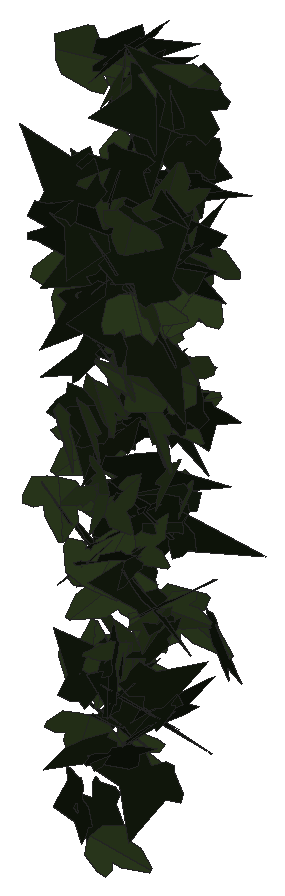
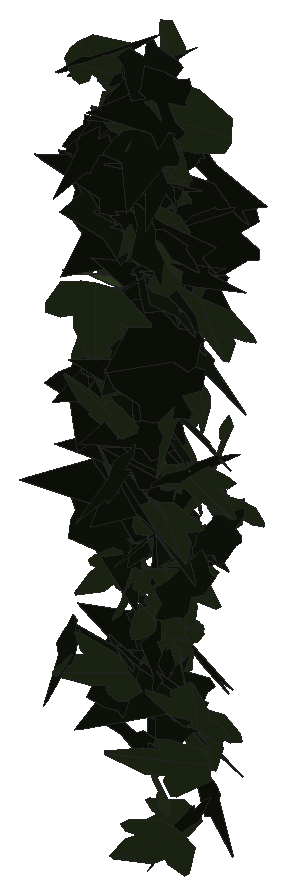
# SketchUp Ruby script. Lengths in inches.
U = 1.inch
M = Sketchup.active_model
def pt(a) = Geom::Point3d.new(a.map { |v| v * U })
def face(e, loops, mat)
  f = e.add_face(loops[0].map { |a| pt(a) })
  loops[1..].each { |l| e.add_face(l.map { |a| pt(a) }).erase! }
  f.material = f.back_material = mat if mat
  f
end
# faces: each face lists its corners as indices into pts; further lists are holes
def faces(e, pts, list, mat = nil) = list.each { |f| face(e, (f[0].is_a?(Array) ? f : [f]).map { |l| l.map { |i| pts[i] } }, mat) }
# xy, xz, yz: faces in a plane at the given z, y or x. An outline is a flat list of corners, or four numbers for a rectangle; further outlines are holes
def ring(l) = l.size == 4 ? [[l[0], l[1]], [l[2], l[1]], [l[2], l[3]], [l[0], l[3]]] : l.each_slice(2).to_a
def flat(e, list, mat, &to3) = list.each { |f| face(e, (f[0].is_a?(Array) ? f : [f]).map { |l| ring(l).map { |u, v| to3.(u, v) } }, mat) }
def xy(e, z, list, mat = nil) = flat(e, list, mat) { |x, y| [x, y, z] }
def xz(e, y, list, mat = nil) = flat(e, list, mat) { |x, z| [x, y, z] }
def yz(e, x, list, mat = nil) = flat(e, list, mat) { |y, z| [x, y, z] }
def lines(e, pts, list) = list.each { |a, b| e.add_line(pt(pts[a]), pt(pts[b])) }
# prism: a flat outline (further loops are holes) pulled along v
def prism(e, loops, v, mat = nil)
  f = face(e, loops, mat); d = Geom::Vector3d.new(v.map { |x| x * U })
  f.pushpull(f.normal.samedirection?(d) ? d.length : -d.length)
end
def box(e, o, s, mat = nil) = prism(e, [[o, [o[0] + s[0], o[1], o[2]], [o[0] + s[0], o[1] + s[1], o[2]], [o[0], o[1] + s[1], o[2]]]], [0, 0, s[2]], mat)
def at(x, y, z, deg = 0) = Geom::Transformation.translation(pt([x, y, z])) * Geom::Transformation.rotation(ORIGIN, Z_AXIS, deg.degrees)
def axes(o, x, y, z) = Geom::Transformation.new([*x, 0, *y, 0, *z, 0, *pt(o).to_a, 1])
def part(name) = M.definitions.add(name)
# library, detail: a bought-in or finely detailed component or shape, given as its bounding box
def library(name, o, s) = part(name).tap { |d| box(d.entities, o, s) }
def detail(e, o, s) = box(e.add_group.entities, o, s)
def put(e, d, t, mat = nil) = e.add_instance(d, t).tap { |i| i.material = mat if mat }
def group(e, t, mat = nil) = e.add_group.tap { |g| g.transformation = t; g.material = mat if mat }.entities
root = M.entities
M.materials.add("1026 AP 7946 SUNNY SIDE UP").color = [254, 231, 186]
M.materials.add("efeu1").color = [18, 25, 13]
M.materials.add("efeu2").color = [43, 57, 29]
c1 = part("ivyleaf_10")
p = [[0,0.5,-0.03],[-0.0625,2.02,-0.43],[-0.19,2.01,-0.46],[-0.54,1.05,-0.29],[-0.52,0.625,-0.18],[-0.83,0.76,-0.28],
  [-1.16,0.64,-0.33],[-1.15,0.33,-0.24],[-0.77,-0.39,0.02],[-0.3,-0.51,0.16],[0.04,-0.48,0.23],[-0.02,2.01,-0.4375],
  [-0.06,2.01,-0.43],[0.04,-0.49,0.23],[0.67,-0.49,0.14],[1.38,0.36,-0.2],[1.375,0.51,-0.24],[0.81,0.65,-0.19],
  [0.62,0.59,-0.15],[0.6,1.09,-0.28],[0.5,1.23,-0.31]]
faces(c1.entities,p,[[0,1,2,3,4,5,6,7,8,9,10],[11,12,0,13,14,15,16,17,18,19,20]],"efeu2")
c2 = part("ivyleaf_9")
p = [[1.54,2.16,1.25],[1.36,2.04,1.19],[-0.21,0.99,0.68],[-0.71,1.11,0.82],[-0.85,0.86,0.67],[-0.8,0.17,0.21],
  [-0.9,-0.01,0.1],[-0.67,-0.16,-0.02],[-0.08,-0.08,-0.05],[-0.03,-0.6,-0.4],[0.65,-0.88,-0.66],[0.83,-0.6,-0.49],
  [1.29,-0.42,-0.43],[1.8125,-0.07,-0.26],[1.21,0.44,0.15]]
faces(c2.entities,p,[[0,1,2,3,4,5,6,7,8,9,10,11,12,13,14]],"efeu1")
put(root,c1,axes([136.21,211.66,278.86],[-0.0278,-0.0094,0.38094],[0.4911,0.19805,0.02172],[-0.31176,0.31282,0.00025]),"1026 AP 7946 SUNNY SIDE UP")
put(root,c2,axes([136.35,211.04,272.625],[0.38727,-0.21719,0.00095],[-0.02228,-0.01932,-0.33751],[0.3408,0.24554,-0.02314]),"1026 AP 7946 SUNNY SIDE UP")
put(root,c1,axes([136.59,210.88,273.87],[-0.17293,0.2877,-0.01409],[-0.00417,-0.0174,-0.31728],[-0.453,-0.10967,0.0083]),"1026 AP 7946 SUNNY SIDE UP")
put(root,c2,axes([137,210.68,277.4375],[-0.06506,0.1165,0.38031],[-0.30524,0.3142,-0.12295],[-0.52547,-0.19694,0.02433]),"1026 AP 7946 SUNNY SIDE UP")
put(root,c1,axes([136.59,211.27,275.9],[0.62304,-0.07737,0.00351],[-0.00388,-0.03262,-0.41475],[0.12175,0.39491,-0.03116]),"1026 AP 7946 SUNNY SIDE UP")
put(root,c1,axes([136.24,212.09,269.64],[0.01205,-0.08359,-0.38142],[0.5698,0.11024,-0.01729],[0.17508,-0.35303,0.08253]),"1026 AP 7946 SUNNY SIDE UP")
put(root,c1,axes([136.81,211.36,273.42],[0.43287,0.00126,-0.17753],[-0.27028,-0.02157,-0.28315],[-0.01967,0.32407,-0.01625]),"1026 AP 7946 SUNNY SIDE UP")
put(root,c2,axes([136.6,211.65,273.69],[-0.15607,-0.3225,0.05031],[-0.00558,-0.05189,-0.34771],[0.51329,-0.09862,0.01152]),"1026 AP 7946 SUNNY SIDE UP")
put(root,c1,axes([136.65,211.44,269.83],[0.56701,-0.03279,0.03863],[-0.0537,0.03854,0.37149],[-0.05731,-0.36051,0.03405]),"1026 AP 7946 SUNNY SIDE UP")
put(root,c1,axes([136.55,210.85,272.87],[0.46298,0.02912,0.08105],[0.12709,-0.02385,-0.30332],[-0.0344,0.3038,-0.02978]),"1026 AP 7946 SUNNY SIDE UP")
put(root,c1,axes([136.84,211.68,274.29],[-0.12414,0.22374,0.25419],[-0.18212,0.21792,-0.24173],[-0.48947,-0.13783,0.02547]),"1026 AP 7946 SUNNY SIDE UP")
put(root,c1,axes([136.53,212.18,268.47],[-0.32013,-0.08956,-0.24599],[0.38005,0.0277,-0.22332],[0.12556,-0.31218,0.04876]),"1026 AP 7946 SUNNY SIDE UP")
put(root,c2,axes([137.02,210.75,268.48],[0.05935,-0.02328,-0.31384],[-0.47182,0.05429,-0.04227],[0.08938,0.302,-0.01476]),"1026 AP 7946 SUNNY SIDE UP")
put(root,c2,axes([136.87,212.02,277.1],[0.06338,0.09978,0.33652],[0.08739,0.32205,-0.10671],[-0.52904,0.06515,0.02269]),"1026 AP 7946 SUNNY SIDE UP")
put(root,c2,axes([137.17,211.42,276.84],[-0.47664,0.02506,-0.15601],[-0.23934,-0.00342,0.31298],[0.03283,0.3389,0.01669]),"1026 AP 7946 SUNNY SIDE UP")
put(root,c2,axes([137.05,210.97,275.02],[-0.30513,0.21423,-0.02605],[0.0044,-0.03314,-0.29725],[-0.33939,-0.19303,0.01957]),"1026 AP 7946 SUNNY SIDE UP")
put(root,c1,axes([136.78,211.96,268.94],[0.31067,-0.25014,0.05999],[-0.03001,0.06076,0.32793],[-0.40323,-0.19724,0.02182]),"1026 AP 7946 SUNNY SIDE UP")
put(root,c1,axes([136.85,211.7,276.52],[0.12673,-0.28952,0.14914],[-0.03583,0.14544,0.31005],[-0.50888,-0.08234,0.01531]),"1026 AP 7946 SUNNY SIDE UP")
put(root,c2,axes([136.95,211.98,278.58],[0.39065,0.09106,-0.21504],[-0.3587,0.09027,-0.23802],[-0.01024,0.31203,0.13374]),"1026 AP 7946 SUNNY SIDE UP")
put(root,c2,axes([137.14,211.5,276.35],[-0.4536,-0.14948,0.15217],[-0.16699,-0.11441,-0.33172],[0.28623,-0.30364,0.04762]),"1026 AP 7946 SUNNY SIDE UP")
put(root,c2,axes([137.27,210.73,270.4],[-0.32936,0.03673,-0.25687],[-0.37724,0.07113,0.21866],[0.12245,0.31794,-0.01726]),"1026 AP 7946 SUNNY SIDE UP")
put(root,c2,axes([137.22,211.02,273.99],[-0.18833,0.21393,0.14502],[-0.16489,0.09937,-0.24905],[-0.36623,-0.15475,0.03755]),"1026 AP 7946 SUNNY SIDE UP")
put(root,c1,axes([136.99,210.89,269.5],[0.45851,0.0798,-0.05094],[-0.11625,0.09365,-0.2902],[-0.09159,0.28062,0.11329]),"1026 AP 7946 SUNNY SIDE UP")
put(root,c2,axes([136.65,211.57,271.76],[0.16872,-0.25415,0.21875],[0.16955,-0.18584,-0.28443],[0.49392,0.15061,0.02291]),"1026 AP 7946 SUNNY SIDE UP")
put(root,c2,axes([136.72,211.74,279],[0.21121,0.10646,0.30666],[0.3911,0.16298,-0.17508],[-0.30537,0.28237,-0.01213]),"1026 AP 7946 SUNNY SIDE UP")
put(root,c2,axes([136.54,210.75,276.83],[0.3807,0.08624,0.32324],[0.48957,0.05017,-0.26183],[-0.14614,0.39274,-0.03508]),"1026 AP 7946 SUNNY SIDE UP")
put(root,c2,axes([137.02,211.08,276.97],[-0.21776,-0.27597,0.09324],[-0.04613,-0.0882,-0.31833],[0.45511,-0.14098,0.01234]),"1026 AP 7946 SUNNY SIDE UP")
put(root,c2,axes([136.93,211.15,268.26],[0.19666,-0.20548,-0.23147],[-0.17736,0.19299,-0.24667],[0.44323,0.16839,0.004]),"1026 AP 7946 SUNNY SIDE UP")
put(root,c2,axes([137.22,211.36,276.01],[-0.34779,0.18257,-0.17716],[-0.17893,0.13283,0.29504],[0.3527,0.24741,-0.02502]),"1026 AP 7946 SUNNY SIDE UP")
put(root,c1,axes([137.17,211.39,275.76],[-0.10162,-0.08496,-0.34058],[-0.20899,-0.30312,0.10541],[-0.49357,0.14584,0.02549]),"1026 AP 7946 SUNNY SIDE UP")
put(root,c2,axes([137.24,211.01,275.89],[-0.00839,0.12717,-0.33309],[-0.00489,-0.3241,-0.13288],[-0.54736,0.00095,0.00629]),"1026 AP 7946 SUNNY SIDE UP")
put(root,c2,axes([137.3125,210.88,269.44],[-0.40724,0.14508,-0.03945],[0.03144,-0.04399,-0.30468],[-0.23417,-0.25821,0.0277]),"1026 AP 7946 SUNNY SIDE UP")
put(root,c2,axes([136.89,211.56,275.63],[0.42135,0.16585,0.0927],[0.14518,0.01918,-0.32296],[-0.25794,0.28172,-0.03035]),"1026 AP 7946 SUNNY SIDE UP")
put(root,c1,axes([137.02,210.83,274.2],[-0.25279,0.2106,-0.11458],[0.08724,-0.09886,-0.27311],[-0.36509,-0.16944,0.01407]),"1026 AP 7946 SUNNY SIDE UP")
put(root,c2,axes([137.28,211.34,276.1875],[-0.16919,0.29544,-0.13858],[0.0653,-0.1298,-0.32464],[-0.50735,-0.11523,0.00443]),"1026 AP 7946 SUNNY SIDE UP")
put(root,c2,axes([137.3,211.63,279.49],[-0.1922,0.29357,-0.15385],[0.05646,-0.14825,-0.32772],[-0.51602,-0.12557,0.02145]),"1026 AP 7946 SUNNY SIDE UP")
put(root,c1,axes([137.32,211.29,272.59],[-0.4199,-0.03014,0.13696],[-0.20203,-0.04319,-0.27585],[0.07241,-0.29524,0.02459]),"1026 AP 7946 SUNNY SIDE UP")
put(root,c1,axes([137.21,211.23,271.65],[0.42787,0.09204,-0.08743],[-0.17297,0.07655,-0.27569],[-0.09515,0.27473,0.10802]),"1026 AP 7946 SUNNY SIDE UP")
put(root,c1,axes([137.13,211.02,274.47],[-0.37343,0.1467,-0.05677],[0.04242,-0.06179,-0.2853],[-0.24319,-0.23603,0.0374]),"1026 AP 7946 SUNNY SIDE UP")
put(root,c1,axes([137.16,210.89,273.06],[-0.24187,-0.22442,-0.06813],[0.07849,0.04429,-0.27956],[0.35883,-0.16095,0.01523]),"1026 AP 7946 SUNNY SIDE UP")
put(root,c2,axes([137.15,211.02,269.72],[0.39357,0.0604,-0.15173],[-0.24928,0.06394,-0.24958],[-0.02762,0.28347,0.09045]),"1026 AP 7946 SUNNY SIDE UP")
put(root,c2,axes([137.33,210.89,272.32],[-0.2468,0.1555,-0.16482],[0.10857,-0.15326,-0.22291],[-0.33465,-0.1644,0.04924]),"1026 AP 7946 SUNNY SIDE UP")
put(root,c1,axes([137.33,211.03,271.64],[0.38389,0.09192,-0.19377],[-0.26093,-0.09249,-0.26826],[-0.20189,0.29432,-0.02173]),"1026 AP 7946 SUNNY SIDE UP")
put(root,c1,axes([137.39,210.7,273.2],[0.14032,-0.20353,-0.31049],[-0.19878,0.27235,-0.22732],[0.53458,0.1547,-0.00303]),"1026 AP 7946 SUNNY SIDE UP")
put(root,c1,axes([137.27,211.84,278.52],[0.51588,0.08091,0.08567],[-0.13834,0.01298,0.34656],[0.11814,-0.3381,0.03172]),"1026 AP 7946 SUNNY SIDE UP")
put(root,c2,axes([136.77,211.66,274.76],[0.27452,-0.01959,0.31551],[0.47403,-0.05567,-0.18097],[0.09123,0.34821,-0.00908]),"1026 AP 7946 SUNNY SIDE UP")
put(root,c2,axes([137.49,211.01,272.21],[-0.06595,0.25632,0.17768],[-0.14759,0.15376,-0.26024],[-0.46148,-0.08581,0.05784]),"1026 AP 7946 SUNNY SIDE UP")
put(root,c2,axes([137.32,211.31,273.99],[-0.42081,0.10903,-0.20635],[0.27057,-0.10758,-0.29689],[-0.23664,-0.31689,0.0275]),"1026 AP 7946 SUNNY SIDE UP")
put(root,c2,axes([137.47,211.1,277.96],[-0.08719,0.05467,-0.46596],[-0.52622,0.30475,0.08194],[0.48682,0.33921,0.00512]),"1026 AP 7946 SUNNY SIDE UP")
put(root,c2,axes([137.14,211.74,277.08],[-0.34262,-0.11414,-0.24567],[0.35966,0.07191,-0.25103],[0.20663,-0.31443,0.02959]),"1026 AP 7946 SUNNY SIDE UP")
put(root,c2,axes([137.32,210.9,272.39],[0.1511,0.23477,0.10943],[0.03974,0.1028,-0.26031],[-0.40236,0.09832,0.01538]),"1026 AP 7946 SUNNY SIDE UP")
put(root,c2,axes([137.09,211.07,276.6],[0.36638,-0.19188,-0.03692],[-0.06325,0.00567,-0.31017],[0.30002,0.23551,-0.02031]),"1026 AP 7946 SUNNY SIDE UP")
put(root,c1,axes([137.3125,211.65,278.96],[-0.00621,0.03652,-0.36529],[-0.07609,-0.35159,-0.03878],[-0.55564,0.04774,0.00939]),"1026 AP 7946 SUNNY SIDE UP")
put(root,c2,axes([137.28,211.52,278.94],[-0.06376,0.19086,-0.30215],[-0.14177,0.28072,0.20193],[0.53313,0.09747,0.01756]),"1026 AP 7946 SUNNY SIDE UP")
put(root,c2,axes([137.04,211.04,275.16],[0.16875,-0.1945,0.19155],[0.13431,-0.16645,-0.22979],[0.40249,0.1371,-0.00363]),"1026 AP 7946 SUNNY SIDE UP")
put(root,c1,axes([137.39,211.55,278.3],[-0.11149,0.29914,0.16396],[-0.13562,0.13955,-0.31232],[-0.51396,-0.10171,0.04685]),"1026 AP 7946 SUNNY SIDE UP")
put(root,c2,axes([137.18,212.26,273.73],[0.33239,-0.21455,-0.14962],[-0.16459,0.09902,-0.30967],[0.37148,0.23584,-0.00333]),"1026 AP 7946 SUNNY SIDE UP")
put(root,c1,axes([137.34,211,270.59],[0.20173,0.26333,-0.13757],[-0.08178,-0.12483,-0.3024],[-0.45808,0.13825,-0.0066]),"1026 AP 7946 SUNNY SIDE UP")
put(root,c2,axes([137.14,211.3,275.8],[0.08792,0.18901,-0.31687],[0.0144,0.31148,0.20003],[0.56892,-0.0371,0.0439]),"1026 AP 7946 SUNNY SIDE UP")
put(root,c2,axes([137.32,210.76,272.11],[0.27843,0.21562,0.03671],[0.05644,0.01495,-0.28674],[-0.33866,0.17977,-0.01761]),"1026 AP 7946 SUNNY SIDE UP")
put(root,c2,axes([137.42,211.0625,270.08],[0.00309,0.03378,0.29174],[-0.23218,-0.24194,0.02939],[0.38331,-0.14682,0.01545]),"1026 AP 7946 SUNNY SIDE UP")
put(root,c2,axes([137.69,210.62,270.75],[-0.01075,0.0115,-0.41567],[-0.5769,0.16825,0.01233],[0.26491,0.36687,0.00998]),"1026 AP 7946 SUNNY SIDE UP")
put(root,c2,axes([137.4375,211.15,270.39],[0.009,-0.03723,0.35175],[0.16453,0.32567,0.03666],[-0.51474,0.10344,0.01787]),"1026 AP 7946 SUNNY SIDE UP")
put(root,c1,axes([137.45,211.03,271.02],[-0.41931,0.16936,0.01898],[-0.04383,-0.01141,-0.32452],[-0.26411,-0.26699,0.02372]),"1026 AP 7946 SUNNY SIDE UP")
put(root,c2,axes([137.52,211.17,275.57],[-0.11185,-0.08103,0.41024],[-0.31525,-0.34518,-0.11115],[0.55662,-0.21178,0.01948]),"1026 AP 7946 SUNNY SIDE UP")
put(root,c1,axes([137.56,211.09,277.75],[-0.24541,-0.33915,0.11256],[-0.0437,-0.10943,-0.38471],[0.5595,-0.1573,0.01932]),"1026 AP 7946 SUNNY SIDE UP")
put(root,c2,axes([137.21,211.25,275.93],[0.04915,-0.01433,0.31361],[0.44985,0.10706,-0.02444],[-0.16549,0.28676,0.02671]),"1026 AP 7946 SUNNY SIDE UP")
put(root,c1,axes([137.59,211.38,276.82],[-0.00173,0.01192,0.34253],[-0.19816,0.30763,-0.00999],[-0.48405,-0.12598,0.00286]),"1026 AP 7946 SUNNY SIDE UP")
put(root,c1,axes([137.62,212.32,276.15],[-0.58236,-0.12129,0.02769],[-0.0225,-0.04448,-0.39986],[0.19428,-0.36872,0.03671]),"1026 AP 7946 SUNNY SIDE UP")
put(root,c1,axes([137.58,210.87,279.4375],[0.07063,-0.29988,-0.16574],[-0.01799,0.15914,-0.31125],[0.53354,0.04506,0.01145]),"1026 AP 7946 SUNNY SIDE UP")
put(root,c2,axes([137.9,211.03,270.04],[-0.43087,0.00792,-0.19862],[-0.29927,0.04458,0.28075],[0.05045,0.3321,-0.03097]),"1026 AP 7946 SUNNY SIDE UP")
put(root,c1,axes([137.37,210.72,271.9375],[0.47829,0.15517,-0.15509],[0.1869,0.09884,0.3509],[0.28512,-0.32509,0.03015]),"1026 AP 7946 SUNNY SIDE UP")
put(root,c1,axes([137.23,211.33,277.73],[0.37309,-0.12489,-0.20168],[0.33213,0.00212,0.26331],[-0.14941,-0.30715,0.08173]),"1026 AP 7946 SUNNY SIDE UP")
put(root,c1,axes([137.62,210.96,270.82],[-0.28703,-0.23804,0.02648],[-0.00293,-0.0326,-0.30865],[0.3767,-0.18163,0.01778]),"1026 AP 7946 SUNNY SIDE UP")
put(root,c1,axes([137.375,210.8,267.91],[0.13366,0.15395,0.2498],[0.14307,0.22446,-0.17901],[-0.42715,0.12336,0.01821]),"1026 AP 7946 SUNNY SIDE UP")
put(root,c2,axes([137.79,210.89,272.27],[-0.35666,0.19229,-0.03783],[0.02219,-0.04166,-0.30571],[-0.30735,-0.22615,0.02183]),"1026 AP 7946 SUNNY SIDE UP")
put(root,c1,axes([137.46,211.33,277.08],[0.50178,0.05428,0.07684],[0.12132,-0.01185,-0.33262],[-0.07878,0.32743,-0.02281]),"1026 AP 7946 SUNNY SIDE UP")
put(root,c2,axes([137.32,211,272.99],[0.43466,-0.02678,0.0877],[0.12816,-0.03829,-0.28478],[0.05771,0.28674,-0.02812]),"1026 AP 7946 SUNNY SIDE UP")
put(root,c2,axes([137.6,210.65,269.41],[0.22054,0.21249,0.03858],[0.03424,0.02905,-0.26211],[-0.33721,0.14192,-0.00139]),"1026 AP 7946 SUNNY SIDE UP")
put(root,c2,axes([137.31,210.95,270.12],[0.72922,-0.0241,-0.0313],[-0.03664,0.11625,-0.46292],[0.04853,0.44997,0.12073]),"1026 AP 7946 SUNNY SIDE UP")
put(root,c1,axes([137.43,210.93,272.95],[0.28832,-0.25183,-0.17037],[0.18268,-0.11771,0.31945],[-0.43576,-0.21597,0.0212]),"1026 AP 7946 SUNNY SIDE UP")
put(root,c2,axes([137.44,211.29,273.93],[0.27042,0.14324,0.21205],[0.25952,0.12194,-0.22968],[-0.29547,0.2382,-0.00767]),"1026 AP 7946 SUNNY SIDE UP")
put(root,c1,axes([137.8,210.87,277.1875],[-0.4575,0.01009,0.08294],[-0.12743,-0.02719,-0.2986],[-0.00384,-0.30065,0.02801]),"1026 AP 7946 SUNNY SIDE UP")
put(root,c1,axes([137.27,212.31,270.74],[0.25936,0.0472,0.32803],[0.48545,0.07702,-0.17622],[-0.1418,0.34999,-0.00328]),"1026 AP 7946 SUNNY SIDE UP")
put(root,c1,axes([137.81,210.79,275.13],[-0.06988,0.18966,0.24115],[-0.16981,0.20971,-0.19584],[-0.44083,-0.11084,0.03721]),"1026 AP 7946 SUNNY SIDE UP")
put(root,c1,axes([137.74,211.4,274.47],[-0.18274,-0.34036,-0.1062],[0.09129,0.08678,-0.36905],[0.55081,-0.1273,0.02593]),"1026 AP 7946 SUNNY SIDE UP")
put(root,c2,axes([137.61,211.56,275.3],[0.27477,-0.23419,-0.18863],[-0.18097,0.14086,-0.30012],[0.42959,0.20913,-0.00578]),"1026 AP 7946 SUNNY SIDE UP")
put(root,c2,axes([137.93,210.79,270.57],[-0.18288,0.25811,-0.06065],[0.02944,-0.05773,-0.29191],[-0.41575,-0.11762,0.00601]),"1026 AP 7946 SUNNY SIDE UP")
put(root,c2,axes([137.77,211.21,274.8],[0.13878,0.22012,0.22107],[0.11532,0.20039,-0.2431],[-0.468,0.11465,0.00565]),"1026 AP 7946 SUNNY SIDE UP")
put(root,c2,axes([137.96,211.32,278.78],[-0.20919,-0.09801,0.34581],[-0.30975,-0.27645,-0.16493],[0.45533,-0.23309,0.04667]),"1026 AP 7946 SUNNY SIDE UP")
put(root,c2,axes([137.46,210.85,278.06],[0.00079,-0.04683,-0.33421],[0.42002,0.18762,-0.0264],[0.29799,-0.26433,0.0381]),"1026 AP 7946 SUNNY SIDE UP")
put(root,c1,axes([138.18,210.82,274.89],[-0.1527,-0.00839,-0.29136],[-0.44447,0.01495,0.09964],[0.01796,0.29861,-0.01142]),"1026 AP 7946 SUNNY SIDE UP")
put(root,c2,axes([137.71,211.76,275.93],[-0.06144,-0.32985,0.0926],[-0.00975,-0.09166,-0.34269],[0.53827,-0.03931,0.00436]),"1026 AP 7946 SUNNY SIDE UP")
put(root,c2,axes([138.22,211.22,272.98],[-0.22459,0.06097,0.25768],[-0.3837,0.05788,-0.15797],[-0.12737,-0.28186,0.0215]),"1026 AP 7946 SUNNY SIDE UP")
put(root,c2,axes([138.23,211.3,277.28],[-0.26503,0.07106,0.25928],[-0.41023,-0.03288,-0.1709],[-0.01778,-0.30078,0.07806]),"1026 AP 7946 SUNNY SIDE UP")
put(root,c2,axes([137.91,211.11,271.8],[0.12554,-0.29697,-0.20202],[0.10043,-0.184,0.31549],[-0.549,-0.10156,0.01152]),"1026 AP 7946 SUNNY SIDE UP")
put(root,c2,axes([137.77,211.07,272.83],[0.29201,0.20854,0.13451],[0.12335,0.1033,-0.28692],[-0.36565,0.20139,0.01063]),"1026 AP 7946 SUNNY SIDE UP")
put(root,c2,axes([137.72,211.31,278.9],[-0.37467,-0.04664,-0.33185],[0.51137,-0.03236,-0.24339],[0.00232,-0.39915,0.05613]),"1026 AP 7946 SUNNY SIDE UP")
put(root,c1,axes([137.63,211.08,272.41],[0.41754,-0.15539,-0.15328],[0.22528,-0.04673,0.31528],[-0.25108,-0.30034,0.02798]),"1026 AP 7946 SUNNY SIDE UP")
put(root,c2,axes([137.87,211.11,269.08],[-0.4321,-0.06833,-0.17831],[0.27359,0.01312,-0.29051],[0.10211,-0.3243,0.02383]),"1026 AP 7946 SUNNY SIDE UP")
put(root,c1,axes([138.15,210.8,276.23],[-0.18183,0.13656,0.27376],[-0.37534,0.12778,-0.17443],[-0.28071,-0.25932,0.05591]),"1026 AP 7946 SUNNY SIDE UP")
put(root,c1,axes([137.76,211.04,275.54],[-0.36973,-0.1488,-0.16393],[0.26124,0.02712,-0.28037],[0.2201,-0.28215,0.05738]),"1026 AP 7946 SUNNY SIDE UP")
put(root,c1,axes([137.96,211.1,271.08],[0.03509,0.29801,-0.15555],[-0.00489,0.1532,0.30848],[0.52649,-0.01844,0.01323]),"1026 AP 7946 SUNNY SIDE UP")
put(root,c2,axes([137.52,211,273.34],[0.30787,0.06908,0.30166],[0.44719,0.07003,-0.2128],[-0.15246,0.34489,-0.01503]),"1026 AP 7946 SUNNY SIDE UP")
put(root,c1,axes([137.77,210.95,275.95],[0.34603,0.27244,0.04558],[0.07042,0.0186,-0.35991],[-0.42786,0.2234,-0.02237]),"1026 AP 7946 SUNNY SIDE UP")
put(root,c1,axes([138.28,211.27,274.91],[0.095,-0.04476,-0.33112],[-0.46752,0.12272,-0.07452],[0.20346,0.30288,-0.01663]),"1026 AP 7946 SUNNY SIDE UP")
put(root,c1,axes([137.87,211.41,279.15],[0.31227,0.23182,0.0206],[0.04093,0.00226,-0.3139],[-0.3634,0.19946,-0.01765]),"1026 AP 7946 SUNNY SIDE UP")
put(root,c2,axes([138.16,211.36,274.6875],[-0.08421,0.29988,-0.0007],[-0.00839,-0.00337,-0.31378],[-0.47147,-0.0535,0.00571]),"1026 AP 7946 SUNNY SIDE UP")
put(root,c2,axes([137.59,211.46,277.43],[0.24691,-0.0527,0.30087],[0.46655,0.04394,-0.15576],[-0.02276,0.32893,0.07102]),"1026 AP 7946 SUNNY SIDE UP")
put(root,c1,axes([137.65,211.78,274.07],[0.31068,-0.09839,-0.25921],[0.39397,-0.04805,0.22226],[-0.15671,-0.31585,0.04486]),"1026 AP 7946 SUNNY SIDE UP")
put(root,c2,axes([137.99,211.14,275.72],[0.28357,-0.07827,-0.22074],[-0.27797,0.12378,-0.19956],[0.22565,0.25084,0.03157]),"1026 AP 7946 SUNNY SIDE UP")
put(root,c2,axes([137.99,211.25,277.06],[0.56329,-0.06479,0.19226],[-0.27576,0.07525,0.37342],[-0.14418,-0.39704,0.03693]),"1026 AP 7946 SUNNY SIDE UP")
put(root,c2,axes([138.25,211.38,276.71],[-0.4007,-0.09096,0.11639],[-0.15092,-0.06687,-0.27761],[0.17184,-0.27083,0.02759]),"1026 AP 7946 SUNNY SIDE UP")
put(root,c2,axes([138.18,210.77,269.97],[-0.10858,0.23587,-0.08253],[0.0123,-0.08243,-0.25321],[-0.39219,-0.06789,0.01491]),"1026 AP 7946 SUNNY SIDE UP")
put(root,c1,axes([138.07,211.47,274.55],[0.4337,-0.12132,-0.05619],[-0.09278,-0.00083,-0.30942],[0.18695,0.28102,-0.02322]),"1026 AP 7946 SUNNY SIDE UP")
put(root,c2,axes([138.36,211.1875,272.88],[-0.06915,-0.00142,-0.29552],[-0.45069,-0.01129,0.04526],[-0.01789,0.28998,0.00202]),"1026 AP 7946 SUNNY SIDE UP")
put(root,c2,axes([138.08,211.18,277.85],[0.27609,0.26329,-0.07708],[-0.0507,-0.07016,-0.32621],[-0.42804,0.17814,-0.01108]),"1026 AP 7946 SUNNY SIDE UP")
put(root,c1,axes([137.9,211.16,274.24],[-0.22338,0.14947,-0.24462],[0.18827,-0.20944,-0.21009],[-0.40024,-0.18194,0.0377]),"1026 AP 7946 SUNNY SIDE UP")
put(root,c2,axes([137.87,211.19,269.8],[0.23426,0.29563,0.02677],[-0.04881,-0.01152,0.34019],[0.46386,-0.15051,0.02228]),"1026 AP 7946 SUNNY SIDE UP")
put(root,c1,axes([138.27,211.6,279.25],[-0.22383,-0.18226,0.2048],[-0.15751,-0.17423,-0.23824],[0.39504,-0.17274,0.02105]),"1026 AP 7946 SUNNY SIDE UP")
put(root,c1,axes([138.14,211.52,274.98],[-0.27106,-0.25903,0.00387],[0.01935,-0.01445,-0.32007],[0.40692,-0.17186,0.01779]),"1026 AP 7946 SUNNY SIDE UP")
put(root,c2,axes([137.9375,210.75,276.54],[-0.30558,0.24601,0.2467],[0.25672,-0.17402,0.32154],[0.47315,0.25331,-0.01513]),"1026 AP 7946 SUNNY SIDE UP")
put(root,c2,axes([138.32,210.88,271.26],[-0.2534,0.21051,-0.01833],[-0.00049,-0.02411,-0.27283],[-0.33235,-0.16046,0.01438]),"1026 AP 7946 SUNNY SIDE UP")
put(root,c2,axes([138.375,211.24,274.42],[0.01957,0.01742,0.32943],[-0.21185,0.29049,-0.00921],[-0.45665,-0.13402,0.01839]),"1026 AP 7946 SUNNY SIDE UP")
put(root,c2,axes([138.26,211.57,277.99],[-0.23351,-0.23375,0.26395],[0.18256,0.23065,0.28599],[-0.51551,0.18756,-0.01828]),"1026 AP 7946 SUNNY SIDE UP")
put(root,c2,axes([137.65,210.99,272.79],[0.18375,0.11541,-0.42326],[0.34355,0.35053,0.16724],[0.57757,-0.24522,0.03518]),"1026 AP 7946 SUNNY SIDE UP")
put(root,c2,axes([138.08,211.51,274.34],[0.37217,0.19214,-0.06031],[-0.04195,-0.06128,-0.31288],[-0.31354,0.23627,-0.02972]),"1026 AP 7946 SUNNY SIDE UP")
put(root,c1,axes([138.18,211.6,275.96],[-0.5002,-0.01917,0.01872],[0.02442,-0.31345,-0.06197],[0.03374,-0.05728,0.32242]),"1026 AP 7946 SUNNY SIDE UP")
put(root,c2,axes([138.15,211.6,277.97],[0.09837,-0.01099,-0.32019],[-0.26631,0.26461,-0.04322],[0.41001,0.17451,0.04875]),"1026 AP 7946 SUNNY SIDE UP")
put(root,c1,axes([138.2,210.875,271.55],[-0.05462,-0.27185,0.04949],[-0.0047,-0.0496,-0.28261],[0.43448,-0.03471,0.00316]),"1026 AP 7946 SUNNY SIDE UP")
put(root,c2,axes([138.18,211.3,276.7],[-0.24328,0.28441,-0.14358],[-0.08046,0.13245,0.33387],[0.49261,0.16209,-0.01638]),"1026 AP 7946 SUNNY SIDE UP")
put(root,c2,axes([137.89,210.9,271.86],[0.27175,-0.23053,0.08536],[0.0777,-0.06815,-0.29721],[0.37799,0.17975,-0.00028]),"1026 AP 7946 SUNNY SIDE UP")
put(root,c2,axes([137.98,211.26,274.46],[0.30819,0.15429,0.15864],[0.21472,0.07301,-0.25544],[-0.26593,0.23776,-0.0224]),"1026 AP 7946 SUNNY SIDE UP")
put(root,c2,axes([138,211.25,276.48],[0.39165,0.1414,0.07162],[0.11317,0.01191,-0.29391],[-0.21977,0.25811,-0.02371]),"1026 AP 7946 SUNNY SIDE UP")
put(root,c2,axes([138.48,211.53,278.93],[-0.22525,-0.32471,-0.02985],[-0.0378,-0.01903,0.36522],[-0.51096,0.14455,-0.01386]),"1026 AP 7946 SUNNY SIDE UP")
put(root,c2,axes([138.1875,212.05,270.82],[0.3096,-0.13371,-0.23577],[-0.31019,0.11507,-0.24424],[0.27681,0.27849,-0.01]),"1026 AP 7946 SUNNY SIDE UP")
put(root,c1,axes([138.27,211.35,273.27],[0.24956,-0.26906,-0.01362],[-0.03051,0.00212,-0.3214],[0.42237,0.15913,-0.01517]),"1026 AP 7946 SUNNY SIDE UP")
put(root,c2,axes([138.36,210.88,270.26],[-0.29346,0.13105,-0.12758],[0.11766,-0.10702,-0.23207],[-0.25883,-0.19723,0.03915]),"1026 AP 7946 SUNNY SIDE UP")
put(root,c2,axes([138.0625,210.82,270.38],[-0.04078,0.00103,0.27428],[0.39333,0.09169,0.02528],[-0.14335,0.25129,-0.00868]),"1026 AP 7946 SUNNY SIDE UP")
put(root,c2,axes([138.48,210.9,271.92],[-0.00978,0.37629,-0.00013],[-0.06263,-0.00291,-0.38554],[-0.58837,-0.00594,0.04104]),"1026 AP 7946 SUNNY SIDE UP")
put(root,c1,axes([138.23,211.05,277.58],[-0.20739,-0.34513,-0.01743],[-0.01145,-0.01323,0.38055],[-0.54308,0.13208,-0.00137]),"1026 AP 7946 SUNNY SIDE UP")
put(root,c1,axes([138.17,211.17,271.52],[-0.13051,-0.14931,-0.24635],[0.22146,0.19297,-0.17397],[0.3827,-0.16258,0.01666]),"1026 AP 7946 SUNNY SIDE UP")
put(root,c1,axes([138.3,211.0625,273.69],[0.0969,-0.2532,0.0998],[0.03627,-0.09557,-0.26902],[0.42554,0.0658,0.0002]),"1026 AP 7946 SUNNY SIDE UP")
put(root,c2,axes([138.14,210.88,275.52],[0.05395,-0.28817,-0.09952],[-0.00704,0.09508,-0.29833],[0.47703,0.03399,0.00685]),"1026 AP 7946 SUNNY SIDE UP")
put(root,c1,axes([138.3125,211.375,277.31],[0.30787,-0.22279,-0.00064],[-0.00841,-0.00556,-0.30548],[0.35021,0.19572,-0.00677]),"1026 AP 7946 SUNNY SIDE UP")
